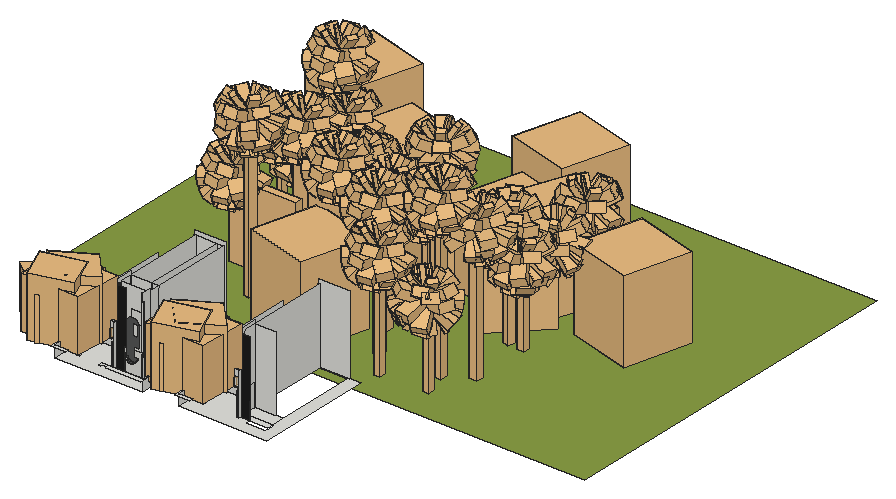
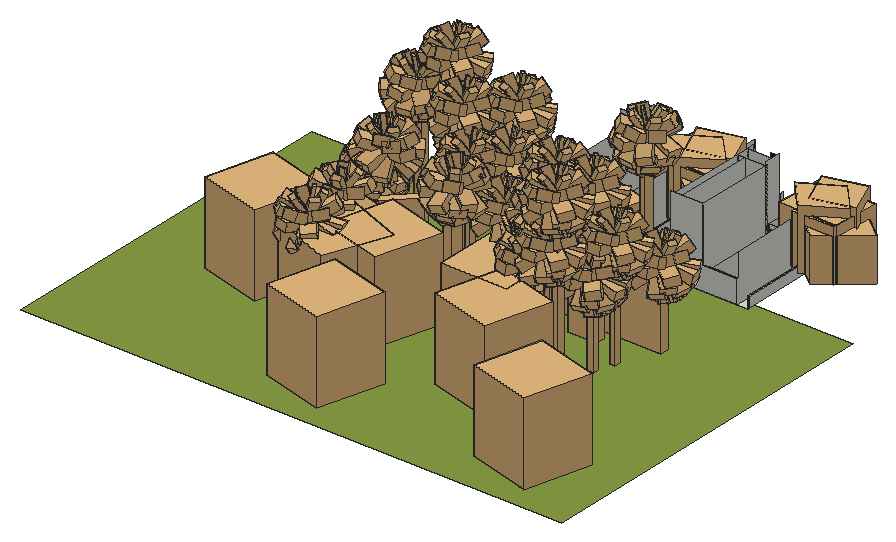
# SketchUp Ruby script. Lengths in inches.
U = 1.inch
M = Sketchup.active_model
def pt(a) = Geom::Point3d.new(a.map { |v| v * U })
def face(e, loops, mat)
  f = e.add_face(loops[0].map { |a| pt(a) })
  loops[1..].each { |l| e.add_face(l.map { |a| pt(a) }).erase! }
  f.material = f.back_material = mat if mat
  f
end
# faces: each face lists its corners as indices into pts; further lists are holes
def faces(e, pts, list, mat = nil) = list.each { |f| face(e, (f[0].is_a?(Array) ? f : [f]).map { |l| l.map { |i| pts[i] } }, mat) }
# xy, xz, yz: faces in a plane at the given z, y or x. An outline is a flat list of corners, or four numbers for a rectangle; further outlines are holes
def ring(l) = l.size == 4 ? [[l[0], l[1]], [l[2], l[1]], [l[2], l[3]], [l[0], l[3]]] : l.each_slice(2).to_a
def flat(e, list, mat, &to3) = list.each { |f| face(e, (f[0].is_a?(Array) ? f : [f]).map { |l| ring(l).map { |u, v| to3.(u, v) } }, mat) }
def xy(e, z, list, mat = nil) = flat(e, list, mat) { |x, y| [x, y, z] }
def xz(e, y, list, mat = nil) = flat(e, list, mat) { |x, z| [x, y, z] }
def yz(e, x, list, mat = nil) = flat(e, list, mat) { |y, z| [x, y, z] }
def lines(e, pts, list) = list.each { |a, b| e.add_line(pt(pts[a]), pt(pts[b])) }
# prism: a flat outline (further loops are holes) pulled along v
def prism(e, loops, v, mat = nil)
  f = face(e, loops, mat); d = Geom::Vector3d.new(v.map { |x| x * U })
  f.pushpull(f.normal.samedirection?(d) ? d.length : -d.length)
end
def box(e, o, s, mat = nil) = prism(e, [[o, [o[0] + s[0], o[1], o[2]], [o[0] + s[0], o[1] + s[1], o[2]], [o[0], o[1] + s[1], o[2]]]], [0, 0, s[2]], mat)
def at(x, y, z, deg = 0) = Geom::Transformation.translation(pt([x, y, z])) * Geom::Transformation.rotation(ORIGIN, Z_AXIS, deg.degrees)
def axes(o, x, y, z) = Geom::Transformation.new([*x, 0, *y, 0, *z, 0, *pt(o).to_a, 1])
def part(name) = M.definitions.add(name)
# library, detail: a bought-in or finely detailed component or shape, given as its bounding box
def library(name, o, s) = part(name).tap { |d| box(d.entities, o, s) }
def detail(e, o, s) = box(e.add_group.entities, o, s)
def put(e, d, t, mat = nil) = e.add_instance(d, t).tap { |i| i.material = mat if mat }
def group(e, t, mat = nil) = e.add_group.tap { |g| g.transformation = t; g.material = mat if mat }.entities
root = M.entities
M.materials.add("COCOLUMBER1").color = [119, 109, 95]
M.materials.add("[Color M06]").color = [84, 84, 84]
M.materials.add("[Color M08]").color = [30, 30, 30]
M.materials.add("[Grass Light Green]").color = [138, 158, 69]
M.materials.add("[Stone_Flagstone_Ashlar]").color = [175, 116, 102]
M.materials.add("[Translucent Glass Safety]").color = [204, 235, 244]
M.materials["[Translucent Glass Safety]"].alpha = 0.5
M.materials.add("[Wood Veneer 01]").color = [120, 70, 37]
c1 = library("Group\#287",[-33.32,-34.9375,32.67],[162.87,159.66,128.34])
c2 = library("Group\#288",[-10.45,-6.67,0],[121.7,116.61,164.95])
c3 = library("Group\#286",[-10.45,-6.67,0],[121.7,116.61,164.95])
c4 = library("Group\#284",[-10.45,-6.67,0],[121.7,116.61,164.95])
c5 = library("Group\#283",[-33.32,-34.9375,32.67],[162.87,159.66,128.34])
c6 = library("Group\#285",[-33.32,-34.9375,81.35],[162.87,159.66,79.66])
c7 = library("Group\#282",[-33.32,-34.9375,77.91],[162.87,159.66,83.1])
c8 = part("Palem Elek")
put(c8.entities,c1,axes([92.2,20.3,-29.73],[0.70711,0.70711,0],[-0.70711,0.70711,0],[0,0,0.91208]))
put(c8.entities,c2,axes([60.27,20.78,0],[1,0,0],[0,1,0],[0,0,0.85762]))
put(c8.entities,c3,at(25.45,60.83,0,-53.5))
put(c8.entities,c4,at(84.4375,135.48,0,-161.4))
put(c8.entities,c5,axes([38.54,105.7,-36.19],[-0.04013,-0.99919,0],[0.99919,-0.04013,0],[0,0,1.11001]))
put(c8.entities,c6,axes([57.15,96.51,-54.45],[-0.02003,-0.49872,0.02965],[0.4996,-0.02007,0],[0.00123,0.03065,0.51628]))
put(c8.entities,c7,axes([74.94,50.39,-54.06],[0.40095,0.29715,0.03075],[-0.29654,0.38966,0.10114],[0.04012,-0.11026,0.54246]))
c9 = part("palem elek\#1")
put(c9.entities,c8,at(-81.14,-74.56,-0.83))
c10 = part("Coqueiro")
put(c10.entities,c9,axes([83.17,89.39,9.5625],[0,1.1016,0],[-1.377,0,0],[0,0,1.39284]))
c11 = library("元件\#5",[-4.39,0,0],[5.37,35.83,90.55])
c12 = part("Group\#3")
g1 = group(c12.entities,at(0,0,0))
xy(g1,0,[[0,0,6,48]],"[Wood Veneer 01]")
xy(g1,4,[[0,4,1.8125,44],[1.8125,4,6,44]])
xy(g1,80,[[0,4,1.8125,44],[1.8125,4,6,44]])
xy(g1,84,[[0,0,6,48]],"[Wood Veneer 01]")
xz(g1,0,[[0,0,6,84]],"[Wood Veneer 01]")
xz(g1,4,[[0,4,1.8125,80],[1.8125,4,6,80]])
xz(g1,44,[[0,4,1.8125,80],[1.8125,4,6,80]])
xz(g1,48,[[0,0,6,84]],"[Wood Veneer 01]")
yz(g1,0,[[[0,0,48,84],[4,4,44,80]]],"[Wood Veneer 01]")
yz(g1,1.8125,[[4,4,44,80]],"[Translucent Glass Safety]")
yz(g1,6,[[[0,0,48,84],[4,4,44,80]]],"[Wood Veneer 01]")
g2 = group(c12.entities,at(0,48,0))
xy(g2,0,[[0,0,6,48]],"[Wood Veneer 01]")
xy(g2,4,[[0,4,1.8125,44],[1.8125,4,6,44]])
xy(g2,80,[[0,4,1.8125,44],[1.8125,4,6,44]])
xy(g2,84,[[0,0,6,48]],"[Wood Veneer 01]")
xz(g2,0,[[0,0,6,84]],"[Wood Veneer 01]")
xz(g2,4,[[0,4,1.8125,80],[1.8125,4,6,80]])
xz(g2,44,[[0,4,1.8125,80],[1.8125,4,6,80]])
xz(g2,48,[[0,0,6,84]],"[Wood Veneer 01]")
yz(g2,0,[[[0,0,48,84],[4,4,44,80]]],"[Wood Veneer 01]")
yz(g2,1.8125,[[4,4,44,80]],"[Translucent Glass Safety]")
yz(g2,6,[[[0,0,48,84],[4,4,44,80]]],"[Wood Veneer 01]")
c13 = library("Palm frond \#1",[-21.27,-0.38,-4.44],[74.64,151.68,26.05])
c14 = part("Palm frond cluster")
put(c14.entities,c13,axes([98.98,59.12,-6.6],[-0.57786,0.81614,0],[-0.81614,-0.57786,0],[0,0,1.8876]))
put(c14.entities,c13,axes([105.83,88.13,9.87],[-0.67944,-0.73373,0],[0.7249,-0.67126,-0.15471],[0.21427,-0.19842,1.86487]))
put(c14.entities,c13,axes([73.46,76.73,-6.83],[1,0,0],[0,0.99443,-0.10543],[0,0.19901,1.87708]))
c15 = part("Palm crown")
put(c15.entities,c13,axes([108.09,116.23,112.23],[0.60444,0.79634,0.02211],[-0.38669,0.31755,-0.86581],[-0.57427,0.42444,0.41215]))
put(c15.entities,c13,axes([136.99,132.05,110.62],[-0.9152,-0.38852,0.10706],[0.08408,-0.44389,-0.89213],[0.32496,-0.66577,0.36188]))
put(c15.entities,c13,axes([122.18,113.8,111.54],[0.08804,0.99481,0.05098],[-0.50379,0.08862,-0.85927],[-0.70852,0.0412,0.41966]))
put(c15.entities,c13,axes([127.99,125.91,114.12],[-0.30715,0.21543,0.04369],[-0.00716,-0.23041,1.0858],[0.26841,0.36655,0.07955]))
put(c15.entities,c13,axes([103.59,126.54,118.32],[0.96893,0.24682,0.01605],[-0.22321,0.84461,0.48663],[0.20112,-0.89679,1.64874]))
put(c15.entities,c13,axes([132.625,118.58,110.86],[-0.79198,0.60227,0.10017],[-0.36651,-0.33776,-0.86694],[-0.4026,-0.59638,0.40255]))
put(c15.entities,c13,axes([132.69,143.375,115.86],[-0.48474,-0.87071,0.083],[0.68927,-0.43869,-0.5766],[1.01639,-0.4196,1.53425]))
put(c15.entities,c14,axes([128.89,9.89,132.21],[0.59014,0.791,-0.16144],[-0.79634,0.60321,0.04452],[0.1326,0.10229,0.98588]))
put(c15.entities,c13,axes([110.58,141.22,117.1],[0.63855,-0.76931,0.0202],[0.63758,0.51415,-0.57371],[0.8135,0.71582,1.54559]))
put(c15.entities,c13,axes([124.78,146.64,115.88],[-0.11221,-0.99112,0.07129],[0.92652,-0.13028,-0.35296],[0.67787,0.04993,1.76097]))
put(c15.entities,c13,axes([122.51,149.42,117.04],[0.39103,-0.91975,0.03404],[0.19966,0.04866,-0.97866],[0.74078,0.32113,0.1671]))
put(c15.entities,c13,axes([109.625,140.35,117.99],[0.86054,-0.50891,0.02211],[0.4462,0.77402,0.44921],[-0.46382,-0.71105,1.68592]))
put(c15.entities,c13,axes([116.71,128.1875,118.1],[0.61604,-0.07661,0.00027],[0.03235,0.25679,-0.96593],[0.09819,0.79033,0.2134]),"COCOLUMBER1")
put(c15.entities,c13,axes([106.79,121.78,118.63],[0.90526,0.41496,-0.09122],[-0.38356,0.70587,-0.59551],[-0.34491,1.08363,1.50659]))
put(c15.entities,c13,axes([127.38,115.49,111.15],[-0.41996,0.90406,0.07938],[-0.48716,-0.15078,-0.8602],[-0.63133,-0.32974,0.41534]))
put(c15.entities,c13,axes([126.87,112.82,117.51],[-0.39428,0.9188,-0.01857],[-0.74747,-0.33238,-0.57517],[-1.00919,-0.40185,1.54373]))
put(c15.entities,c13,axes([136.51,114.68,116.54],[-0.8132,0.57038,0.11567],[-0.44883,-0.74115,0.49924],[0.69933,0.66833,1.62089]))
put(c15.entities,c13,axes([139.34,132.85,114.96],[-0.95658,-0.27018,0.10937],[0.1925,-0.86734,-0.45898],[0.41314,-0.78901,1.66428]))
put(c15.entities,c13,axes([114.58,111.42,117.76],[0.273,0.96044,0.05495],[-0.82871,0.20578,0.52048],[0.92224,-0.35418,1.60843]))
put(c15.entities,c14,axes([34.06,50.17,99.19],[1,0,0],[0,0.96593,0.25882],[0,-0.25882,0.96593]))
put(c15.entities,c13,axes([129.57,143.93,113.7],[-0.59821,-0.79634,0.08934],[0.41703,-0.40458,-0.81388],[0.56418,-0.37071,0.47337]))
put(c15.entities,c13,axes([130.72,144.4375,116.95],[-0.38164,-0.91976,0.09155],[0.8496,-0.31006,0.42666],[-0.68716,0.45418,1.6984]))
put(c15.entities,c13,axes([131.04,111.78,119.35],[-0.80044,0.5994,0.00413],[-0.42618,-0.56425,-0.7071],[-0.79563,-1.07169,1.33472]))
put(c15.entities,c13,axes([110.2,144.05,126.35],[0.60643,-0.7943,0.03632],[0.64903,0.52087,0.55448],[-0.86705,-0.59022,1.56936]))
put(c15.entities,c13,axes([142.64,131.42,116.29],[-0.95847,-0.25692,0.12379],[0.28487,-0.84195,0.45823],[-0.02548,0.8956,1.66141]))
put(c15.entities,c13,axes([119.45,118.27,117.33],[0.21648,0.59293,0.03228],[-0.46829,0.12335,0.87492],[0.90601,-0.35995,0.53567]))
put(c15.entities,c13,axes([117.27,113.7,118.04],[0.23506,0.97049,-0.05375],[-0.80388,0.16302,-0.57201],[-1.03133,0.33537,1.54496]))
put(c15.entities,c13,axes([111.15,130.86,117.79],[0.59448,-0.21434,0.01115],[0.17045,0.51639,0.83922],[-0.32671,-0.8747,0.60458]))
put(c15.entities,c13,axes([131.22,120.64,116.67],[-0.51397,0.3605,0.07311],[-0.2051,-0.46687,0.86021],[0.60585,0.75173,0.55245]))
put(c15.entities,c13,axes([124.93,138.67,117.02],[-0.21153,-0.59293,0.0562],[0.56288,-0.12335,0.81728],[-0.84066,0.35995,0.63331]))
put(c15.entities,c13,axes([125.97,109.88,116.19],[-0.24621,0.96375,0.10281],[-0.94431,-0.21463,-0.24942],[-0.41209,-0.29916,1.81761]))
put(c15.entities,c13,axes([112.49,114.18,118.67],[0.68775,0.72163,-0.07906],[-0.67912,0.60109,-0.4213],[-0.48416,0.64828,1.70539]))
c16 = part("Group\#111")
put(c16.entities,c15,axes([-0.04,31.24,176.27],[0.54092,-0.14494,0],[0.14494,0.54092,0],[0,0,0.56]),"[Stone_Flagstone_Ashlar]")
g3 = group(c16.entities,at(43.85,611.85,9.84))
detail(g3,[29.01,-534.03,-9.84],[20.18,17.89,236.22])
c17 = library("Group\#103",[280.3,-607.43,-9.84],[21.76,21.76,393.7])
c18 = part("Group\#14")
put(c18.entities,c15,axes([14.65,13.97,332.76],[0.56,0,0],[0,0.56,0],[0,0,0.56]),"[Stone_Flagstone_Ashlar]")
put(c18.entities,c17,at(-205.96,691.71,9.84))
c19 = library("Group\#102",[336.49,-607.32,-9.84],[23.63,23.62,472.44])
c20 = part("Group\#12")
put(c20.entities,c15,axes([14.65,13.97,408.41],[0.56,0,0],[0,0.56,0],[0,0,0.56]),"[Stone_Flagstone_Ashlar]")
put(c20.entities,c19,axes([-199.25,630.26,9.84],[0.8099,0,0],[0,0.92,0],[0,0,1]))
c21 = part("Group\#13")
put(c21.entities,c15,axes([14.65,13.97,257.21],[0.56,0,0],[0,0.56,0],[0,0,0.56]),"[Stone_Flagstone_Ashlar]")
g4 = group(c21.entities,at(-87.26,634.75,9.84))
detail(g4,[163.83,-557.35,-9.84],[17.02,18.12,316.37])
c22 = library("Coconut",[0,0,0],[6,6,6])
c23 = part("Group\#106")
detail(c23.entities,[126.53,-566.4375,-31.76],[21.43,21.47,314.96])
c24 = part("Group\#109")
put(c24.entities,c15,axes([14.65,13.97,253.0625],[0.56,0,0],[0,0.56,0],[0,0,0.56]),"[Stone_Flagstone_Ashlar]")
put(c24.entities,c23,at(-54.86,642.08,31.76))
c25 = library("Group\#349",[-31.7,-22.28,0],[197.44,197.48,245.38])
c26 = library("Group\#217",[-86.05,-583.93,-9.84],[105.44,25.13,372.44])
c27 = part("Group\#229")
put(c27.entities,c15,axes([14.65,13.97,296.01],[0.56,0,0],[0,0.56,0],[0,0,0.56]),"[Stone_Flagstone_Ashlar]")
put(c27.entities,c26,axes([86.81,656.51,9.45],[1,0,0],[0,1,0],[0,0,0.96]))
c28 = library("Group\#220",[-509.61,-583,-9.84],[198.33,25,224.95])
c29 = part("Group\#226")
put(c29.entities,c15,axes([14.65,13.97,164.57],[0.56,0,0],[0,0.56,0],[0,0,0.56]),"[Stone_Flagstone_Ashlar]")
put(c29.entities,c28,at(588.97,655.37,9.84))
c30 = library("Group\#218",[-201.8,-584.81,-9.84],[84.72,26.88,386.61])
c31 = library("Group\#219",[-284.02,-582.12,-9.84],[34.81,21.51,275.59])
c32 = part("LANDSCAPING+Coconut+Trees")
xy(c32.entities,0,[[-341.57,-22.89,1280.875,1071.24]],"[Grass Light Green]")
put(c32.entities,c16,at(644.25,162.65,0.08,-90))
put(c32.entities,c18,at(534.68,153.22,0.24))
put(c32.entities,c20,at(627.57,68.88,0.24))
g5 = group(c32.entities,at(441.06,62.32,0.24))
put(g5,c15,axes([14.65,13.97,334.3],[0.56,0,0],[0,0.56,0],[0,0,0.56]),"[Stone_Flagstone_Ashlar]")
g6 = group(g5,at(-161.71,683.51,9.84))
detail(g6,[235.77,-605.36,-9.84],[21.85,21.73,393.32])
put(c32.entities,c21,at(507.45,-17.04,0.04))
g7 = group(c32.entities,at(384.92,163.75,0.52))
put(g7,c15,axes([14.65,13.97,253.0625],[0.56,0,0],[0,0.56,0],[0,0,0.56]),"[Stone_Flagstone_Ashlar]")
put(g7,c22,axes([78.15,82.49,296.44],[0.8993,1.53487,-0.03138],[-1.51998,0.89531,0.23158],[0.21557,-0.09025,1.76378]))
put(g7,c22,axes([79.68,82.54,287.24],[0.80142,1.36782,-0.02796],[-1.35455,0.79787,0.20637],[0.1921,-0.08042,1.57182]))
put(g7,c22,axes([77.51,71.8,291.02],[0.8993,1.53487,-0.03138],[-1.51998,0.89531,0.23158],[0.21557,-0.09025,1.76378]))
put(g7,c22,axes([86.52,87.55,293.71],[1.04679,1.7866,-0.03652],[-1.76927,1.04215,0.26956],[0.25092,-0.10505,2.05306]))
put(g7,c22,axes([92.01,70.93,291.34],[1.26662,2.16178,-0.04419],[-2.14081,1.261,0.32616],[0.30361,-0.12711,2.4842]))
put(g7,c23,at(-54.86,642.08,31.76))
put(c32.entities,c24,at(322.43,275.42,0.52,75))
put(c32.entities,c25,at(215.66,444.05,0))
put(c32.entities,c27,at(219.87,194.55,1.28))
put(c32.entities,c29,at(-99.86,200.06,0.67))
g8 = group(c32.entities,at(71.46,249.51,0.63))
put(g8,c15,axes([14.65,13.97,325.99],[0.56,0,0],[0,0.56,0],[0,0,0.56]),"[Stone_Flagstone_Ashlar]")
put(g8,c30,at(259.05,660.06,9.84))
g9 = group(c32.entities,at(290.4,300.18,0.67))
put(g9,c15,axes([14.65,13.97,214.81],[0.56,0,0],[0,0.56,0],[0,0,0.56]),"[Stone_Flagstone_Ashlar]")
put(g9,c31,at(354.13,659.23,9.84))
put(c32.entities,c25,at(768.63,688.84,0,159))
put(c32.entities,c25,at(573.53,797.54,0,75))
put(c32.entities,c20,at(18.43,450.01,0.24))
put(c32.entities,c18,at(864.55,292.18,0.24,180))
put(c32.entities,c16,at(695.7,287.05,0.08))
put(c32.entities,c16,at(135.65,408.5625,0.08))
put(c32.entities,c29,at(771.29,622.71,0.67,-134.5))
put(c32.entities,c16,at(664.4,571.51,0.08))
put(c32.entities,c27,at(563.8125,499.28,1.28,140.1))
put(c32.entities,c21,at(450.29,232.17,0.04))
put(c32.entities,c21,at(-49.04,312.68,0.04))
put(c32.entities,c21,at(52.82,431.375,0.04))
put(c32.entities,c25,at(259.5,238.44,0,-105))
put(c32.entities,c25,at(533.19,658.43,0,-105))
put(c32.entities,c16,at(-26.35,370.51,0.08))
put(c32.entities,c25,at(-48.71,797.54,0,75))
put(c32.entities,c25,at(238.42,585.39,0,75))
put(c32.entities,c25,at(891.93,658.43,0,-105))
put(c32.entities,c20,at(220.5,234.49,0.24,165))
put(c32.entities,c24,at(795.86,275.42,0.52,75))
xy(root,6.125,[[[516.89,908.02,979.81,908.02,979.81,1529.04,572.21,1529.04,572.21,1130.875,690.69,1130.875,690.69,1088.75,700.74,1088.75,700.74,1095.9375,747.92,1095.9375,747.92,1088.75,767.84,1088.75,767.84,1097.28,709.53,1097.28,709.53,1139.4,579.44,1139.4,579.44,1521.81,916.04,1521.81,916.04,1027.17,922.83,1027.17,922.83,983.34,921.96,983.34,921.96,971.36,820.52,971.36,820.52,983.34,820.02,983.34,820.02,996.48,770.9,996.48,770.9,983.34,759.32,983.34,759.32,1088.75,747.92,1088.75,747.92,1095.9375,700.74,1095.9375,700.74,1088.75,690.69,1088.75,690.69,1130.875,572.21,1130.875,572.21,1529.04,516.89,1529.04],[572.21,985.23,585.21,996.48]],[[1172.39,908.02,1635.31,908.02,1635.31,1529.04,1227.71,1529.04,1227.71,1130.875,1346.19,1130.875,1346.19,1088.75,1356.24,1088.75,1356.24,1095.9375,1403.42,1095.9375,1403.42,1088.75,1423.34,1088.75,1423.34,1097.28,1365.03,1097.28,1365.03,1139.4,1234.94,1139.4,1234.94,1521.81,1571.54,1521.81,1571.54,1027.17,1578.33,1027.17,1578.33,983.34,1577.46,983.34,1577.46,971.36,1476.02,971.36,1476.02,983.34,1475.52,983.34,1475.52,996.48,1426.4,996.48,1426.4,983.34,1414.82,983.34,1414.82,1088.75,1403.42,1088.75,1403.42,1095.9375,1356.24,1095.9375,1356.24,1088.75,1346.19,1088.75,1346.19,1130.875,1227.71,1130.875,1227.71,1529.04,1172.39,1529.04],[1227.71,985.23,1240.71,996.48]],[820.52,971.36,916.04,971.36,916.04,983.34,915.16,983.34,915.16,992.96,820.52,992.96],[759.32,983.34,770.9,996.48],[820.02,983.34,820.52,993.35],
  [915.16,983.34,916.04,993.35],[916.04,983.34,922.83,993.35],[1414.82,983.34,1426.4,996.48],[572.21,985.23,585.21,996.48],[1227.71,985.23,1240.71,996.48],
  [820.52,992.96,915.16,993.35],[[820.52,993.35,916.04,993.35,916.04,1097.28,767.84,1097.28,767.84,1088.75,759.32,1088.75,759.32,1003.71,780.56,1003.71,780.56,996.48,820.52,996.48],[767.84,1012.23,769.03,1088.75]],[820.52,993.35,820.52,996.48,780.56,996.48,780.56,1003.71,769.03,1003.71,769.03,1027.17,916.04,1027.17,916.04,993.35],[820.52,993.35,820.52,996.48,780.56,996.48,780.56,1003.71,820.52,1003.71,820.52,996.48,916.04,996.48,916.04,993.35],[820.02,993.35,820.52,996.48],
  [916.04,993.35,922.83,996.48],[759.32,996.48,770.9,1003.71],[820.52,996.48,820.52,1003.71,769.03,1003.71,769.03,1027.17,916.04,1027.17,916.04,996.48],[770.9,996.48,780.56,1003.71],[916.04,996.48,922.83,1027.17],
  [1414.82,996.48,1426.4,1003.71],[1476.02,996.48,1476.02,1003.71,1424.53,1003.71,1424.53,1027.17,1571.54,1027.17,1571.54,996.48],[1426.4,996.48,1436.06,1003.71],[759.32,1003.71,759.32,1088.75,767.84,1088.75,767.84,1012.23,769.03,1012.23,769.03,1003.71],[1414.82,1003.71,1414.82,1088.75,1423.34,1088.75,1423.34,1012.23,1424.53,1012.23,1424.53,1003.71],
  [767.84,1012.23,769.03,1088.75],[1423.34,1012.23,1424.53,1088.75],[769.03,1027.17,916.04,1028.46],[769.03,1028.46,916.04,1028.46,916.04,1097.28,767.84,1097.28,767.84,1089.96,769.03,1089.96],[1424.53,1028.46,1571.54,1028.46,1571.54,1097.28,1423.34,1097.28,1423.34,1089.96,1424.53,1089.96],
  [767.84,1088.75,769.03,1089.96],[1423.34,1088.75,1424.53,1089.96],[709.53,1097.28,767.84,1521.81],[767.84,1097.28,879.04,1521.81],[879.04,1097.28,916.04,1521.81],
  [1365.03,1097.28,1423.34,1521.81],[579.44,1139.4,709.53,1521.81],[1234.94,1139.4,1365.03,1521.81]])
xy(root,40.13,[[608.18,1130.875,655.81,1139.4],[1263.68,1130.875,1311.31,1139.4]])
xy(root,66.125,[[508.71,889.52,588.18,889.52,588.18,908.02,516.89,908.02,516.89,1529.04,508.71,1529.04],[762.97,889.52,776.1,889.52,776.1,895.77,800.41,895.77,800.41,889.52,986.33,889.52,986.33,1529.04,979.81,1529.04,979.81,908.02,762.97,908.02],[1164.21,889.52,1243.68,889.52,1243.68,908.02,1172.39,908.02,1172.39,1529.04,1164.21,1529.04]])
xz(root,983.34,[[759.32,6.125,770.9,132.47],[915.16,6.125,916.04,126.125],[916.04,6.125,921.96,126.125],[921.96,6.125,922.83,6.125,922.83,421.25,916.04,421.25,916.04,141.26,921.96,141.26],[1414.82,6.125,1426.4,132.47]])
xz(root,985.23,[[572.21,6.125,585.21,128.75],[1227.71,6.125,1240.71,128.75]])
xz(root,986.55,[[[865.7,73.1,873.41,74.12,874.67,74.64,879.76,76.75,880.59,77.09,886.6,81.7,886.76,81.83,888.28,83.8125,891.49,88,891.8125,88.77,892.69,90.875,894.47,95.18,894.55,95.83,894.74,97.27,870.3,97.27,870.3,145.27,895.48,145.27,895.48,253.3125,894.83,258.27,894.55,260.375,894.47,261.02,892.69,265.33,891.8125,267.4375,891.49,268.21,888.28,272.39,886.76,274.375,886.6,274.5,880.59,279.11,879.76,279.45,874.67,281.5625,873.41,282.09,865.7,283.1,857.99,282.09,856.72,281.5625,851.63,279.45,850.8,279.11,844.79,274.5,844.63,274.375,843.11,272.39,839.9,268.21,839.58,267.4375,838.71,265.33,836.92,261.02,836.84,260.375,836.56,258.27,835.91,253.3125,835.91,102.89,836.56,97.9375,836.84,95.83,836.92,95.18,838.71,90.875,839.58,88.77,839.9,88,843.11,83.8125,844.63,81.83,844.79,81.7,850.8,77.09,851.63,76.75,856.72,74.64,857.99,74.12],[868.14,196.89,894.83,258.27]]],"[Color M06]")
xz(root,993.35,[[820.02,6.125,820.52,8.32],[820.52,6.125,907.49,8.32],[907.49,6.125,915.16,8.32],[915.16,6.125,916.04,8.32],[916.04,6.125,922.83,8.32],
  [1475.52,6.125,1476.02,8.32],[820.02,8.32,820.52,95.62],[820.52,8.32,907.49,126.125],[907.49,8.32,915.16,109.9375],[915.16,8.32,916.04,109.9375],
  [1475.52,8.32,1476.02,95.62]])
xz(root,996.48,[[572.21,6.125,585.21,128.75],[1227.71,6.125,1240.71,128.75]])
xz(root,996.48,[[770.9,6.125,820.02,6.125,820.02,126.125,820.52,126.125,820.52,402.64,780.56,402.64,780.56,226.8,770.9,226.8],[1426.4,6.125,1475.52,6.125,1475.52,126.125,1476.02,126.125,1476.02,402.64,1436.06,402.64,1436.06,226.8,1426.4,226.8]],"[Color M08]")
xz(root,1003.71,[[769.03,6.125,770.9,126.125],[770.9,6.125,780.56,126.125],[1424.53,6.125,1426.4,126.125],[1426.4,6.125,1436.06,126.125]])
xz(root,1012.23,[[767.84,6.125,769.03,402.64],[1423.34,6.125,1424.53,402.64]])
xz(root,1028.46,[[[769.03,6.125,916.04,402.64],[820.52,226.8,913.34,295.72]]])
xz(root,1088.75,[[690.69,6.125,700.74,6.125,700.74,101.1875,747.92,101.1875,747.92,6.125,759.32,6.125,759.32,126.125,690.69,126.125],[759.32,6.125,769.03,126.125],[1346.19,6.125,1356.24,6.125,1356.24,101.1875,1403.42,101.1875,1403.42,6.125,1414.82,6.125,1414.82,126.125,1346.19,126.125],[1414.82,6.125,1424.53,126.125]])
xz(root,1089.96,[[767.84,6.125,769.03,402.64],[1423.34,6.125,1424.53,402.64]])
xz(root,1095.9375,[[700.74,6.125,747.92,101.1875],[1356.24,6.125,1403.42,101.1875]])
xz(root,1097.28,[[767.84,6.125,879.04,402.64],[879.04,6.125,916.04,402.64],[1423.34,6.125,1534.54,402.64]])
xz(root,1130.875,[[[572.21,6.125,690.69,126.125],[608.18,40.13,655.81,95.51]],[[1227.71,6.125,1346.19,126.125],[1263.68,40.13,1311.31,95.51]]])
xz(root,1139.4,[[579.44,6.125,587.96,126.125],[[587.96,6.125,709.53,126.125],[608.18,40.13,655.81,95.51]],[1234.94,6.125,1243.46,126.125],[[1243.46,6.125,1365.03,126.125],[1263.68,40.13,1311.31,95.51]]])
xz(root,1521.81,[[579.44,6.125,709.53,126.125],[709.53,6.125,709.53,126.125,759.32,126.125,759.32,402.64,767.84,402.64,767.84,6.125],[767.84,6.125,879.04,402.64],[879.04,6.125,916.04,402.64],[1234.94,6.125,1365.03,126.125],
  [1365.03,6.125,1365.03,126.125,1414.82,126.125,1414.82,402.64,1423.34,402.64,1423.34,6.125]])
xz(root,1529.04,[[508.71,6.125,516.89,66.125],[572.21,6.125,572.21,126.125,759.32,126.125,759.32,421.25,922.83,421.25,922.83,6.125],[979.81,6.125,986.33,66.125],[1164.21,6.125,1172.39,66.125],[1227.71,6.125,1227.71,126.125,1414.82,126.125,1414.82,421.25,1578.33,421.25,1578.33,6.125]])
yz(root,516.89,[[908.02,6.125,1529.04,66.125]])
yz(root,572.21,[[985.23,6.125,985.23,128.75,989.28,128.75,989.28,126.125,996.48,126.125,996.48,6.125],[1130.875,6.125,1130.875,252.47,1521.81,252.47,1521.81,126.125,1529.04,126.125,1529.04,6.125]])
yz(root,579.44,[[1139.4,6.125,1521.81,126.125]])
yz(root,585.21,[[985.23,6.125,996.48,128.75]])
yz(root,608.18,[[1130.875,40.13,1139.4,95.51]])
yz(root,655.81,[[1130.875,40.13,1139.4,95.51]])
yz(root,690.69,[[1088.75,6.125,1130.875,126.125]])
yz(root,700.74,[[1088.75,6.125,1095.9375,101.1875]])
yz(root,709.53,[[1097.28,6.125,1139.4,126.125],[1139.4,6.125,1521.81,126.125]])
yz(root,747.92,[[1088.75,6.125,1095.9375,101.1875]])
yz(root,759.32,[[983.34,6.125,983.34,132.47,996.48,132.47,996.48,126.125,1088.75,126.125,1088.75,6.125]])
yz(root,767.84,[[1012.23,6.125,1012.23,421.25,1097.28,421.25,1097.28,402.64,1089.96,402.64,1089.96,6.125],[1089.96,6.125,1097.28,402.64],[1097.28,6.125,1521.81,402.64]])
yz(root,769.03,[[1003.71,6.125,1012.23,126.125],[1012.23,6.125,1027.17,126.125],[1027.17,6.125,1028.46,126.125],[1028.46,6.125,1088.75,126.125],[1088.75,6.125,1089.96,6.125,1089.96,402.64,1028.46,402.64,1028.46,126.125,1088.75,126.125]])
yz(root,770.9,[[983.34,6.125,996.48,226.8]])
yz(root,820.02,[[993.35,6.125,996.48,8.32],[993.35,8.32,996.48,95.62]])
yz(root,879.04,[[1097.28,6.125,1521.81,402.64]])
yz(root,915.16,[[983.34,6.125,993.35,126.125]])
yz(root,916.04,[[993.35,6.125,1028.46,402.64],[1028.46,6.125,1097.28,402.64],[1097.28,6.125,1521.81,402.64]])
yz(root,922.83,[[983.34,6.125,1027.17,6.125,1027.17,421.25,983.34,421.25,983.34,376.875,993.35,376.875,993.35,109.9375,990,109.9375,985.91,110.21,983.34,110.72]])
yz(root,979.81,[[908.02,6.125,1529.04,66.125]])
yz(root,1172.39,[[908.02,6.125,1529.04,66.125]])
yz(root,1227.71,[[985.23,6.125,985.23,128.75,989.28,128.75,989.28,126.125,996.48,126.125,996.48,6.125],[1130.875,6.125,1130.875,252.47,1521.81,252.47,1521.81,126.125,1529.04,126.125,1529.04,6.125]])
yz(root,1234.94,[[1139.4,6.125,1521.81,126.125]])
yz(root,1240.71,[[985.23,6.125,996.48,128.75]])
yz(root,1263.68,[[1130.875,40.13,1139.4,95.51]])
yz(root,1311.31,[[1130.875,40.13,1139.4,95.51]])
yz(root,1346.19,[[1088.75,6.125,1130.875,126.125]])
yz(root,1356.24,[[1088.75,6.125,1095.9375,101.1875]])
yz(root,1365.03,[[1097.28,6.125,1139.4,126.125],[1139.4,6.125,1521.81,126.125]])
yz(root,1403.42,[[1088.75,6.125,1095.9375,101.1875]])
yz(root,1414.82,[[983.34,6.125,983.34,132.47,996.48,132.47,996.48,126.125,1088.75,126.125,1088.75,6.125]])
yz(root,1423.34,[[1012.23,6.125,1012.23,421.25,1097.28,421.25,1097.28,402.64,1089.96,402.64,1089.96,6.125],[1089.96,6.125,1097.28,402.64],[1097.28,6.125,1521.81,402.64]])
yz(root,1424.53,[[1003.71,6.125,1012.23,126.125],[1012.23,6.125,1027.17,126.125],[1027.17,6.125,1028.46,126.125],[1028.46,6.125,1088.75,126.125],[1088.75,6.125,1089.96,6.125,1089.96,402.64,1028.46,402.64,1028.46,126.125,1088.75,126.125]])
yz(root,1426.4,[[983.34,6.125,996.48,226.8]])
yz(root,1475.52,[[993.35,6.125,996.48,8.32],[993.35,8.32,996.48,95.62]])
p = [[857.99,986.55,74.12],[857.99,971.36,74.12],[865.7,971.36,73.1],[865.7,986.55,73.1],[873.41,971.36,74.12],[873.41,986.55,74.12],
  [856.72,986.55,74.64],[856.72,972.36,74.64],[856.72,971.36,74.64],[874.67,971.36,74.64],[874.67,972.36,74.64],[874.67,986.55,74.64],
  [851.63,972.36,76.75],[851.63,986.55,76.75],[879.76,972.36,76.75],[879.76,986.55,76.75],[850.8,986.55,77.09],[850.8,971.36,77.09],
  [851.63,971.36,76.75],[879.76,971.36,76.75],[880.59,971.36,77.09],[880.59,986.55,77.09],[886.6,971.36,81.7],[886.6,972.36,81.7],
  [886.6,986.55,81.7],[844.63,972.36,81.83],[844.79,972.36,81.7],[844.79,986.55,81.7],[844.63,986.55,81.83],[886.76,972.36,81.83],
  [886.76,986.55,81.83],[843.11,972.36,83.8125],[843.11,986.55,83.8125],[888.28,972.36,83.8125],[888.28,986.55,83.8125],[888.28,971.36,83.8125],
  [891.49,971.36,88],[891.49,986.55,88],[891.8125,971.36,88.77],[891.8125,972.36,88.77],[891.8125,986.55,88.77],[838.71,972.36,90.875],
  [839.58,972.36,88.77],[839.58,986.55,88.77],[838.71,986.55,90.875],[892.69,972.36,90.875],[892.69,986.55,90.875],[820.52,1003.71,24.125],
  [820.52,1003.71,6.125],[820.52,1012.23,24.125]]
faces(root,p,[[0,1,2,3],[3,2,4,5],[6,7,8,1,0],[5,4,9,10,11],[12,7,6,13],[10,14,15,11],[16,17,18,12,13],[15,14,19,20,21],
  [21,20,22,23,24],[25,26,27,28],[23,29,30,24],[31,25,28,32],[29,33,34,30],[34,33,35,36,37],[37,36,38,39,40],[41,42,43,44],
  [39,45,46,40]],"[Color M06]")
lines(root,p,[[47,48],[47,49]])
put(root,c10,axes([319.13,937.64,29.13],[1.38444,0,0],[0,1.38444,0],[0,0,1.38444]))
put(root,c10,axes([974.63,937.64,29.13],[1.38444,0,0],[0,1.38444,0],[0,0,1.38444]))
put(root,c11,axes([700.74,1089.14,6.11],[0,-1.05,0],[1.302,0,0],[0,0,1.05]))
put(root,c11,axes([1356.24,1089.14,6.11],[0,-1.05,0],[1.302,0,0],[0,0,1.05]))
put(root,c12,axes([608.18,1133.76,40.13],[0,-0.48,0],[0.49609,0,0],[0,0,0.65923]))
put(root,c12,axes([1263.68,1133.76,40.13],[0,-0.48,0],[0.49609,0,0],[0,0,0.65923]))
put(root,c32,axes([600.99,1519.5,0],[1.7595,0,0],[0,1.7595,0],[0,0,1.7595]))
